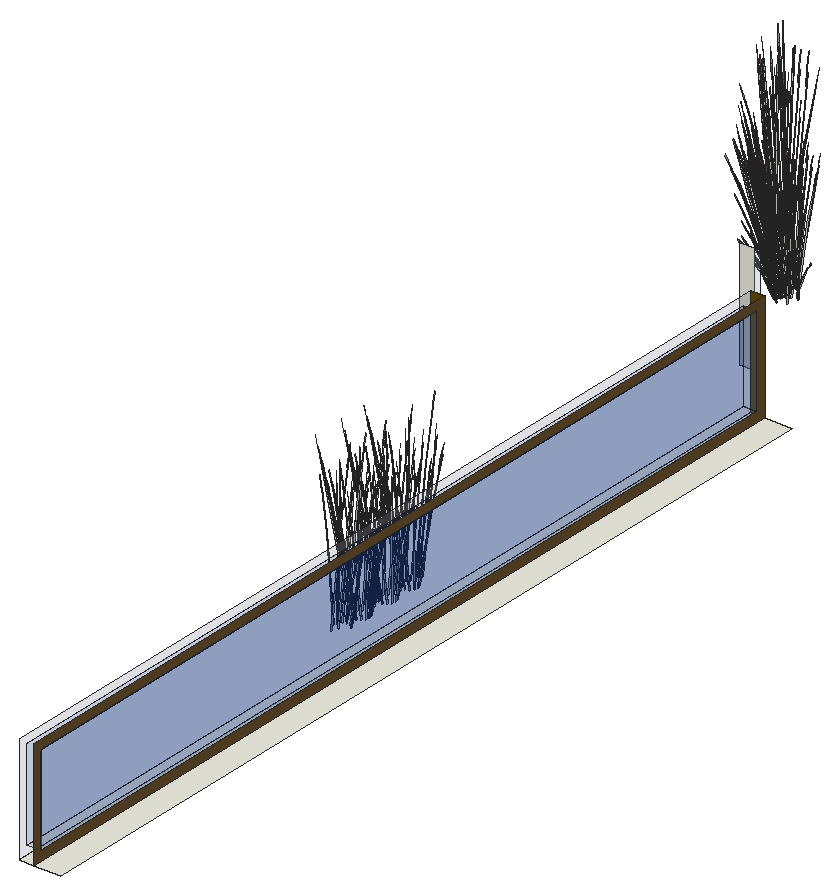
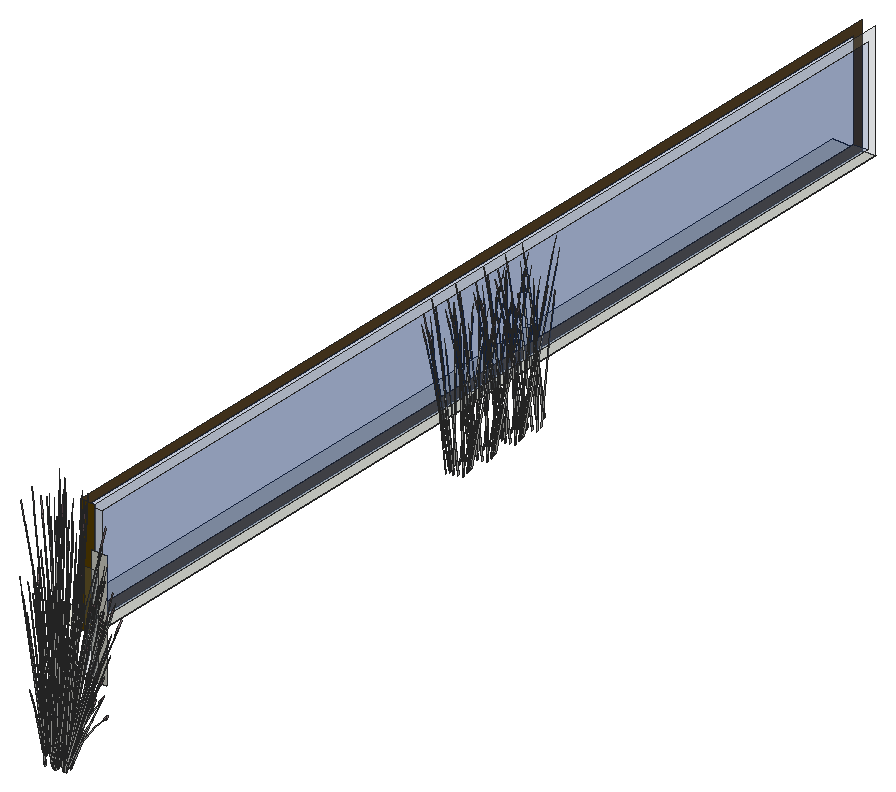
# SketchUp Ruby script. Lengths in inches.
U = 1.inch
M = Sketchup.active_model
def pt(a) = Geom::Point3d.new(a.map { |v| v * U })
def face(e, loops, mat)
  f = e.add_face(loops[0].map { |a| pt(a) })
  loops[1..].each { |l| e.add_face(l.map { |a| pt(a) }).erase! }
  f.material = f.back_material = mat if mat
  f
end
# faces: each face lists its corners as indices into pts; further lists are holes
def faces(e, pts, list, mat = nil) = list.each { |f| face(e, (f[0].is_a?(Array) ? f : [f]).map { |l| l.map { |i| pts[i] } }, mat) }
# xy, xz, yz: faces in a plane at the given z, y or x. An outline is a flat list of corners, or four numbers for a rectangle; further outlines are holes
def ring(l) = l.size == 4 ? [[l[0], l[1]], [l[2], l[1]], [l[2], l[3]], [l[0], l[3]]] : l.each_slice(2).to_a
def flat(e, list, mat, &to3) = list.each { |f| face(e, (f[0].is_a?(Array) ? f : [f]).map { |l| ring(l).map { |u, v| to3.(u, v) } }, mat) }
def xy(e, z, list, mat = nil) = flat(e, list, mat) { |x, y| [x, y, z] }
def xz(e, y, list, mat = nil) = flat(e, list, mat) { |x, z| [x, y, z] }
def yz(e, x, list, mat = nil) = flat(e, list, mat) { |y, z| [x, y, z] }
def lines(e, pts, list) = list.each { |a, b| e.add_line(pt(pts[a]), pt(pts[b])) }
# prism: a flat outline (further loops are holes) pulled along v
def prism(e, loops, v, mat = nil)
  f = face(e, loops, mat); d = Geom::Vector3d.new(v.map { |x| x * U })
  f.pushpull(f.normal.samedirection?(d) ? d.length : -d.length)
end
def box(e, o, s, mat = nil) = prism(e, [[o, [o[0] + s[0], o[1], o[2]], [o[0] + s[0], o[1] + s[1], o[2]], [o[0], o[1] + s[1], o[2]]]], [0, 0, s[2]], mat)
def at(x, y, z, deg = 0) = Geom::Transformation.translation(pt([x, y, z])) * Geom::Transformation.rotation(ORIGIN, Z_AXIS, deg.degrees)
def axes(o, x, y, z) = Geom::Transformation.new([*x, 0, *y, 0, *z, 0, *pt(o).to_a, 1])
def part(name) = M.definitions.add(name)
# library, detail: a bought-in or finely detailed component or shape, given as its bounding box
def library(name, o, s) = part(name).tap { |d| box(d.entities, o, s) }
def detail(e, o, s) = box(e.add_group.entities, o, s)
def put(e, d, t, mat = nil) = e.add_instance(d, t).tap { |i| i.material = mat if mat }
def group(e, t, mat = nil) = e.add_group.tap { |g| g.transformation = t; g.material = mat if mat }.entities
root = M.entities
M.materials.add("D01_Frost_White").color = [238, 238, 227]
M.materials.add("D08_Bronzed_Mustard").color = [102, 74, 0]
M.materials.add("Glass_Basic_01").color = [161, 173, 186]
M.materials["Glass_Basic_01"].alpha = 0.25
M.materials.add("Glass_Sky Reflection_01").color = [0, 46, 142]
M.materials["Glass_Sky Reflection_01"].alpha = 0.25
M.materials.add("LightPink_Translucent").color = [144, 107, 117]
M.materials["LightPink_Translucent"].alpha = 0.75
M.materials.add("Wood_Veneer_15_1K").color = [103, 79, 44]
c1 = part("blade")
p = [[2.15,0.21,22],[0,0.17,0],[0.09,0.45,0],[2.18,0.31,22],[2.29,0.31,22],[0.38,0.45,0],
  [2.48,0.24,33],[2.49,0.24,33],[2.48,0.22,33]]
faces(c1.entities,p,[[0,1,2,3],[4,5,2,3],[6,3,4,7],[8,0,3,6]])
c2 = part("seeds")
p = [[0.3,-0.1,1.38],[-0.01,-0.03,1.59],[-0.01,-0.03,0.03],[0.14,-0.07,-0.07],[0.29,-0.03,3],[0.15,0.01,3.11]]
faces(c2.entities,p,[[0,1,2,3],[1,0,4,5]],"LightPink_Translucent")
c3 = part("blade with seeds")
put(c3.entities,c1,at(0,0,0))
put(c3.entities,c2,axes([2.4,0.25,30.99],[1.5799,-0.05474,1.17369],[-0.12525,1.92788,0.29478],[-0.07173,-0.02425,1.56792]))
xy(root,156,[[439,373,442,574.02],[442,373,448,574.02]],"D01_Frost_White")
xy(root,158,[[439,375,442,572.02]],"Glass_Basic_01")
xz(root,572.02,[[439,158,442,178]],"Glass_Basic_01")
xz(root,574.02,[[439,156,442,180]],"D08_Bronzed_Mustard")
xz(root,586,[[427,156,430,180]],"D01_Frost_White")
xz(root,588,[[427,158,430,178]],"Glass_Basic_01")
yz(root,439,[[[373,156,574.02,180],[375,158,572.02,178]]],"Glass_Basic_01")
yz(root,439,[[375,158,572.02,178]],"Glass_Sky Reflection_01")
yz(root,442,[[375,158,572.02,178]],"Glass_Sky Reflection_01")
yz(root,442,[[[373,156,574.02,180],[375,158,572.02,178]]],"Wood_Veneer_15_1K")
put(root,c3,axes([429.26,472.51,154.77],[0.28319,-0.27058,-0.05481],[0.25948,0.29635,-0.2485],[0.01827,0.08397,0.81966]))
put(root,c3,axes([428.77,471.52,154.28],[-0.4038,-0.12331,0.45013],[0.13808,-0.40538,0.37115],[0.02427,0.15942,0.93144]))
put(root,c3,axes([427.46,473.45,154.27],[0.34057,0.13158,0.29918],[-0.09933,0.38387,-0.38624],[-0.13712,0.0352,0.73904]))
put(root,c3,axes([428.4,477.19,154.3],[0.45651,-0.12123,0.45419],[0.07923,0.47555,0.3745],[-0.10736,-0.14016,0.93983]))
put(root,c3,axes([430.36,474.97,154.27],[-0.23317,-0.29531,0.29918],[0.26625,-0.27955,-0.38624],[0.13527,0.04253,0.73904]))
put(root,c3,axes([429.43,477.58,154.27],[-0.12355,0.36271,0.29918],[-0.36044,-0.10579,-0.38624],[-0.03305,-0.14603,0.73904]))
put(root,c3,axes([430.21,477.99,154.27],[-0.27728,0.24833,0.29918],[-0.26248,-0.28355,-0.38624],[0.03994,-0.14407,0.73904]))
put(root,c3,axes([427.52,474.37,154.27],[0.35672,-0.06741,0.29918],[0.09419,0.38534,-0.38624],[-0.10222,0.1035,0.73904]))
put(root,c3,axes([428.56,477.64,154.27],[0.06329,0.37991,0.29918],[-0.36182,0.10032,-0.38624],[-0.09718,-0.10887,0.73904]))
put(root,c3,axes([427.48,477.89,154.3],[0.33843,-0.34808,0.45419],[0.29188,0.36965,0.3745],[-0.15878,-0.06421,0.93983]))
put(root,c3,axes([426.71,475.46,154.77],[0.36162,0.1259,-0.05481],[-0.11124,0.3875,-0.2485],[-0.05915,0.05883,0.81966]))
put(root,c3,axes([429.64,475.48,154.27],[-0.06329,-0.37991,0.29918],[0.36182,-0.10032,-0.38624],[0.09718,0.10887,0.73904]))
put(root,c3,axes([430.6875,478.76,154.27],[-0.35672,0.06741,0.29918],[-0.09419,-0.38534,-0.38624],[0.10222,-0.1035,0.73904]))
put(root,c3,axes([428,475.14,154.27],[0.27728,-0.24833,0.29918],[0.26248,0.28355,-0.38624],[-0.03994,0.14407,0.73904]))
put(root,c3,axes([428.78,475.54,154.27],[0.12355,-0.36271,0.29918],[0.36044,0.10579,-0.38624],[0.03305,0.14603,0.73904]))
put(root,c3,axes([427.84,478.15,154.27],[0.23317,0.29531,0.29918],[-0.26625,0.27955,-0.38624],[-0.13527,-0.04253,0.73904]))
put(root,c3,axes([429.26,476.84,154.77],[0.28319,-0.27058,-0.05481],[0.25948,0.29635,-0.2485],[0.01827,0.08397,0.81966]))
put(root,c3,axes([428.77,475.84,154.28],[-0.4038,-0.12331,0.45013],[0.13808,-0.40538,0.37115],[0.02427,0.15942,0.93144]))
put(root,c3,axes([430.75,479.68,154.27],[-0.34057,-0.13158,0.29918],[0.09933,-0.38387,-0.38624],[0.13712,-0.0352,0.73904]))
put(root,c3,axes([427.46,478.98,154.27],[0.34057,0.13158,0.29918],[-0.09933,0.38387,-0.38624],[-0.13712,0.0352,0.73904]))
put(root,c3,axes([430.36,480.51,154.27],[-0.23317,-0.29531,0.29918],[0.26625,-0.27955,-0.38624],[0.13527,0.04253,0.73904]))
put(root,c3,axes([427.52,479.9,154.27],[0.35672,-0.06741,0.29918],[0.09419,0.38534,-0.38624],[-0.10222,0.1035,0.73904]))
put(root,c3,axes([428.4,484.41,154.3],[0.45651,-0.12123,0.45419],[0.07923,0.47555,0.3745],[-0.10736,-0.14016,0.93983]))
put(root,c3,axes([426.71,481,154.77],[0.36162,0.1259,-0.05481],[-0.11124,0.3875,-0.2485],[-0.05915,0.05883,0.81966]))
put(root,c3,axes([429.64,481.02,154.27],[-0.06329,-0.37991,0.29918],[0.36182,-0.10032,-0.38624],[0.09718,0.10887,0.73904]))
put(root,c3,axes([429.43,484.79,154.27],[-0.12355,0.36271,0.29918],[-0.36044,-0.10579,-0.38624],[-0.03305,-0.14603,0.73904]))
put(root,c3,axes([430.21,485.2,154.27],[-0.27728,0.24833,0.29918],[-0.26248,-0.28355,-0.38624],[0.03994,-0.14407,0.73904]))
put(root,c3,axes([428,480.67,154.27],[0.27728,-0.24833,0.29918],[0.26248,0.28355,-0.38624],[-0.03994,0.14407,0.73904]))
put(root,c3,axes([428.78,481.08,154.27],[0.12355,-0.36271,0.29918],[0.36044,0.10579,-0.38624],[0.03305,0.14603,0.73904]))
put(root,c3,axes([428.56,484.85,154.27],[0.06329,0.37991,0.29918],[-0.36182,0.10032,-0.38624],[-0.09718,-0.10887,0.73904]))
put(root,c3,axes([427.48,485.1,154.3],[0.33843,-0.34808,0.45419],[0.29188,0.36965,0.3745],[-0.15878,-0.06421,0.93983]))
put(root,c3,axes([429.26,482.375,154.77],[0.28319,-0.27058,-0.05481],[0.25948,0.29635,-0.2485],[0.01827,0.08397,0.81966]))
put(root,c3,axes([428.77,481.38,154.28],[-0.4038,-0.12331,0.45013],[0.13808,-0.40538,0.37115],[0.02427,0.15942,0.93144]))
put(root,c3,axes([430.6875,485.97,154.27],[-0.35672,0.06741,0.29918],[-0.09419,-0.38534,-0.38624],[0.10222,-0.1035,0.73904]))
put(root,c3,axes([427.84,485.37,154.27],[0.23317,0.29531,0.29918],[-0.26625,0.27955,-0.38624],[-0.13527,-0.04253,0.73904]))
put(root,c3,axes([430.75,486.89,154.27],[-0.34057,-0.13158,0.29918],[0.09933,-0.38387,-0.38624],[0.13712,-0.0352,0.73904]))
put(root,c3,axes([427.46,486.2,154.27],[0.34057,0.13158,0.29918],[-0.09933,0.38387,-0.38624],[-0.13712,0.0352,0.73904]))
put(root,c3,axes([428.4,490.57,154.3],[0.45651,-0.12123,0.45419],[0.07923,0.47555,0.3745],[-0.10736,-0.14016,0.93983]))
put(root,c3,axes([430.36,487.72,154.27],[-0.23317,-0.29531,0.29918],[0.26625,-0.27955,-0.38624],[0.13527,0.04253,0.73904]))
put(root,c3,axes([429.43,490.96,154.27],[-0.12355,0.36271,0.29918],[-0.36044,-0.10579,-0.38624],[-0.03305,-0.14603,0.73904]))
put(root,c3,axes([427.52,487.12,154.27],[0.35672,-0.06741,0.29918],[0.09419,0.38534,-0.38624],[-0.10222,0.1035,0.73904]))
put(root,c3,axes([430.21,491.37,154.27],[-0.27728,0.24833,0.29918],[-0.26248,-0.28355,-0.38624],[0.03994,-0.14407,0.73904]))
put(root,c3,axes([426.71,488.21,154.77],[0.36162,0.1259,-0.05481],[-0.11124,0.3875,-0.2485],[-0.05915,0.05883,0.81966]))
put(root,c3,axes([428.56,491.02,154.27],[0.06329,0.37991,0.29918],[-0.36182,0.10032,-0.38624],[-0.09718,-0.10887,0.73904]))
put(root,c3,axes([429.64,488.23,154.27],[-0.06329,-0.37991,0.29918],[0.36182,-0.10032,-0.38624],[0.09718,0.10887,0.73904]))
put(root,c3,axes([427.48,491.27,154.3],[0.33843,-0.34808,0.45419],[0.29188,0.36965,0.3745],[-0.15878,-0.06421,0.93983]))
put(root,c3,axes([428,487.89,154.27],[0.27728,-0.24833,0.29918],[0.26248,0.28355,-0.38624],[-0.03994,0.14407,0.73904]))
put(root,c3,axes([430.6875,492.14,154.27],[-0.35672,0.06741,0.29918],[-0.09419,-0.38534,-0.38624],[0.10222,-0.1035,0.73904]))
put(root,c3,axes([428.78,488.29,154.27],[0.12355,-0.36271,0.29918],[0.36044,0.10579,-0.38624],[0.03305,0.14603,0.73904]))
put(root,c3,axes([429.26,489.59,154.77],[0.28319,-0.27058,-0.05481],[0.25948,0.29635,-0.2485],[0.01827,0.08397,0.81966]))
put(root,c3,axes([428.77,488.59,154.28],[-0.4038,-0.12331,0.45013],[0.13808,-0.40538,0.37115],[0.02427,0.15942,0.93144]))
put(root,c3,axes([427.84,491.53,154.27],[0.23317,0.29531,0.29918],[-0.26625,0.27955,-0.38624],[-0.13527,-0.04253,0.73904]))
put(root,c3,axes([430.75,493.06,154.27],[-0.34057,-0.13158,0.29918],[0.09933,-0.38387,-0.38624],[0.13712,-0.0352,0.73904]))
put(root,c3,axes([427.46,492.36,154.27],[0.34057,0.13158,0.29918],[-0.09933,0.38387,-0.38624],[-0.13712,0.0352,0.73904]))
put(root,c3,axes([430.36,493.89,154.27],[-0.23317,-0.29531,0.29918],[0.26625,-0.27955,-0.38624],[0.13527,0.04253,0.73904]))
put(root,c3,axes([427.52,493.28,154.27],[0.35672,-0.06741,0.29918],[0.09419,0.38534,-0.38624],[-0.10222,0.1035,0.73904]))
put(root,c3,axes([426.71,494.38,154.77],[0.36162,0.1259,-0.05481],[-0.11124,0.3875,-0.2485],[-0.05915,0.05883,0.81966]))
put(root,c3,axes([429.64,494.4,154.27],[-0.06329,-0.37991,0.29918],[0.36182,-0.10032,-0.38624],[0.09718,0.10887,0.73904]))
put(root,c3,axes([428,494.05,154.27],[0.27728,-0.24833,0.29918],[0.26248,0.28355,-0.38624],[-0.03994,0.14407,0.73904]))
put(root,c3,axes([428.78,494.46,154.27],[0.12355,-0.36271,0.29918],[0.36044,0.10579,-0.38624],[0.03305,0.14603,0.73904]))
put(root,c3,axes([429.26,495.75,154.77],[0.28319,-0.27058,-0.05481],[0.25948,0.29635,-0.2485],[0.01827,0.08397,0.81966]))
put(root,c3,axes([428.77,494.76,154.28],[-0.4038,-0.12331,0.45013],[0.13808,-0.40538,0.37115],[0.02427,0.15942,0.93144]))
put(root,c3,axes([416.2,609.51,156.77],[0.09368,0.15143,1.44779],[-0.43286,0.12749,0.11706],[-0.09783,-0.23774,0.61892]))
put(root,c3,axes([416.91,608.5,157.48],[-0.06268,-0.06613,1.47793],[-0.4183,0.04193,-0.23373],[-0.06676,-0.15817,0.11853]))
put(root,c3,axes([417.88,609.29,155.68],[-0.11649,0.09547,1.20808],[-0.34886,-0.1671,-0.25981],[0.06467,-0.20781,0.51652]))
put(root,c3,axes([417.35,609.62,157.7],[-0.19559,-0.38351,-0.60019],[0.40262,-0.21373,0.07243],[-0.04574,-0.1853,0.84903]))
put(root,c3,axes([416.08,609.11,155.68],[-0.02482,0.15429,1.20808],[-0.36278,0.12916,-0.25981],[-0.0848,-0.19943,0.51652]))
put(root,c3,axes([417.02,608.77,154.75],[-0.06874,0.01699,1.48974],[-0.38012,-0.19128,-0.22758],[0.00638,-0.15955,0.25375]))
put(root,c3,axes([418.17,609.99,157.7],[0.01066,-0.43628,-0.60019],[0.44902,0.0293,0.07243],[0.04739,-0.18483,0.84903]))
put(root,c3,axes([418.79,609.3125,157.48],[-0.00396,-0.09387,1.47793],[-0.33411,-0.2713,-0.23373],[0.05166,-0.16446,0.11853]))
put(root,c3,axes([417.39,609.29,157.32],[0.12355,-0.36271,-0.29918],[0.36044,0.10579,0.38624],[-0.03305,-0.14603,0.73904]))
put(root,c3,axes([417.66,609.77,156.77],[-0.0763,0.16212,1.44779],[-0.3201,-0.3355,0.11706],[0.1444,-0.2091,0.61892]))
put(root,c3,axes([418.7,608.97,157.47],[-0.04162,0.03603,1.49853],[-0.40776,-0.12155,-0.1416],[-0.01476,-0.15722,0.26519]))
put(root,c3,axes([417.21,609.54,157.45],[-0.40284,-0.11824,-0.43168],[0.13808,-0.40538,-0.33437],[-0.03694,-0.16321,0.82598]))
put(root,c3,axes([417.46,608.53,155.83],[0.05257,0.27504,0.97034],[-0.29163,-0.15233,0.71294],[0.03138,-0.14083,0.21373]))
put(root,c3,axes([418.08,609.85,157.45],[-0.29336,-0.31691,-0.43168],[0.3099,-0.27755,-0.33437],[0.04464,-0.16102,0.82598]))
put(root,c3,axes([416.49,608.28,157.47],[-0.00765,0.05653,1.49853],[-0.37706,0.20517,-0.1416],[-0.11096,-0.10488,0.26519]))
put(root,c3,axes([416.4,609.29,157.8],[0.45651,-0.12123,0.45419],[0.07923,0.47555,0.3745],[-0.10736,-0.14016,0.93983]))
put(root,c3,axes([417.43,609.375,157.49],[0.4038,0.12331,0.40553],[-0.13808,0.40538,0.33437],[-0.02427,-0.15942,0.83914]))
put(root,c3,axes([417.55,609.52,157.75],[-0.40102,0.2196,-0.10273],[-0.19707,-0.38974,-0.57019],[-0.05291,-0.16424,0.8664]))
put(root,c3,axes([418.38,610.02,157.75],[-0.45039,-0.02337,-0.10273],[0.01231,-0.44247,-0.57019],[0.03129,-0.17041,0.8664]))
put(root,c3,axes([418.35,609.73,157.32],[0.27728,-0.24833,-0.29918],[0.26248,0.28355,0.38624],[0.03994,-0.14407,0.73904]))
put(root,c3,axes([415.96,608.86,155.83],[0.21377,0.16416,0.97034],[-0.31132,0.09868,0.71294],[-0.06661,-0.12616,0.21373]))
put(root,c3,axes([417.54,609.35,157.49],[0.30197,-0.1603,0.05432],[0.1478,0.29231,0.42765],[-0.02916,-0.12885,0.65209]))
put(root,c3,axes([416.47,609.73,157.7],[-0.34944,-0.22798,-0.60019],[0.24834,-0.39949,0.07243],[-0.1266,-0.13612,0.84903]))
put(root,c3,axes([416.35,609.43,157.32],[-0.06329,-0.37991,-0.29918],[0.36182,-0.10032,0.38624],[-0.09718,-0.10887,0.73904]))
put(root,c3,axes([416.51,609.39,157.49],[0.18625,-0.29962,0.05432],[0.26523,0.17444,0.42765],[-0.08575,-0.09606,0.65209]))
put(root,c3,axes([415.79,609.35,154.75],[-0.0397,0.06213,1.48974],[-0.40116,0.13396,-0.22758],[-0.09691,-0.12186,0.25375]))
put(root,c3,axes([415.57,609.98,156.77],[0.15222,0.08126,1.44779],[-0.31502,0.34091,0.11706],[-0.19634,-0.15379,0.61892]))
put(root,c3,axes([418.7,609.58,154.75],[-0.06134,-0.03716,1.48974],[-0.15755,-0.41512,-0.22758],[0.10629,-0.11265,0.25375]))
put(root,c3,axes([417.43,609.67,157.76],[-0.12355,0.36271,0.29918],[-0.36044,-0.10579,-0.38624],[-0.03305,-0.14603,0.73904]))
put(root,c3,axes([416.31,609.74,157.45],[-0.40438,0.11212,-0.43168],[-0.07074,-0.4246,-0.33437],[-0.10862,-0.12168,0.82598]))
put(root,c3,axes([418.35,609.83,157.49],[0.29182,0.32181,0.40553],[-0.3099,0.27755,0.33437],[0.05383,-0.15098,0.83914]))
put(root,c3,axes([416.59,609.36,158.08],[-0.2735,0.45217,-0.11506],[-0.39608,-0.2605,-0.63862],[-0.13768,-0.12775,0.97037]))
put(root,c3,axes([418.46,609.86,157.49],[0.33677,0.02198,0.05432],[-0.00923,0.33185,0.42765],[0.03524,-0.12712,0.65209]))
put(root,c3,axes([418.21,610.08,157.76],[-0.27728,0.24833,0.29918],[-0.26248,-0.28355,-0.38624],[0.03994,-0.14407,0.73904]))
put(root,c3,axes([418.7,610.75,157.7],[0.21406,-0.37215,-0.60019],[0.37511,0.26448,0.07243],[0.12781,-0.13483,0.84903]))
put(root,c3,axes([416.38,609.67,155.5],[-0.25622,-0.47263,0],[0.42866,-0.26357,-0.43598],[0.09763,-0.06003,1.38303]))
put(root,c3,axes([418.6875,610.58,157.45],[-0.10528,-0.43067,-0.43168],[0.39868,-0.07534,-0.33437],[0.11425,-0.11568,0.82598]))
put(root,c3,axes([416.95,609.1,155.29],[-0.28319,0.27058,-0.03288],[-0.25948,-0.29635,-0.1491],[-0.01827,-0.08397,0.4918]))
put(root,c3,axes([415.54,609.23,157.48],[-0.08817,-0.00333,1.47793],[-0.28072,0.33293,-0.23373],[-0.14978,-0.06803,0.11853]))
put(root,c3,axes([418.875,610.89,157.75],[-0.37908,-0.26007,-0.10273],[0.21839,-0.37663,-0.57019],[0.1071,-0.13092,0.8664]))
put(root,c3,axes([417.31,612.31,156.3],[0.35414,0.19019,1.27785],[-0.34693,0.40974,0.50532],[-0.1554,-0.24285,1.07126]))
put(root,c3,axes([416.56,609.74,157.76],[0.06329,0.37991,0.29918],[-0.36182,0.10032,-0.38624],[-0.09718,-0.10887,0.73904]))
put(root,c3,axes([415.46,610.99,155.2],[0,-0.47166,-0.41945],[0.45849,0,0],[0,-0.10742,1.33059]))
put(root,c3,axes([416.73,609.6,155.2],[0.38354,-0.23583,-0.41945],[0.22925,0.42288,0],[0.08735,-0.05371,1.33059]))
put(root,c3,axes([419.01,610.41,155.68],[-0.1464,-0.01397,1.20808],[-0.14998,-0.37477,-0.25981],[0.17985,-0.10602,0.51652]))
put(root,c3,axes([415.48,609.98,157.8],[0.33843,-0.34808,0.45419],[0.29188,0.36965,0.3745],[-0.15878,-0.06421,0.93983]))
put(root,c3,axes([419.81,610.77,157.47],[-0.05353,-0.00358,1.49853],[-0.22227,-0.38383,-0.1416],[0.08926,-0.1262,0.26519]))
put(root,c3,axes([419.18,609.72,155.83],[-0.1365,0.2401,0.97034],[-0.11733,-0.32258,0.71294],[0.11274,-0.08083,0.21373]))
put(root,c3,axes([418.98,610.625,157.32],[0.35672,-0.06741,-0.29918],[0.09419,0.38534,0.38624],[0.10222,-0.1035,0.73904]))
put(root,c3,axes([415.63,609.98,157.49],[0.02064,-0.35866,0.05432],[0.3116,0.00983,0.42765],[-0.11936,-0.03753,0.65209]))
put(root,c3,axes([416.7,611.18,155.36],[0.19883,-0.425,-0.37796],[0.41314,0.20454,0.1819],[0,-0.09797,1.2135]))
put(root,c3,axes([415.51,610.09,157.32],[-0.23317,-0.29531,-0.29918],[0.26625,-0.27955,0.38624],[-0.13527,-0.04253,0.73904]))
put(root,c3,axes([416.89,610.97,155.75],[-0.04775,-0.53819,-0.2458],[0.49736,-0.03254,-0.42242],[0.08758,-0.07169,1.34921]))
put(root,c3,axes([415.65,611,155.21],[0.28606,-0.29428,-0.2617],[0.28606,0.29428,0.2617],[0,-0.09479,1.17405]))
put(root,c3,axes([415.54,609.59,155.29],[-0.11822,0.38513,-0.03288],[-0.36385,-0.11847,-0.1491],[-0.05524,-0.06299,0.4918]))
put(root,c3,axes([418.6875,610.85,157.76],[-0.35672,0.06741,0.29918],[-0.09419,-0.38534,-0.38624],[0.10222,-0.1035,0.73904]))
put(root,c3,axes([416.66,611.54,155.75],[-0.46151,-0.22505,-0.2458],[0.22222,-0.475,-0.42242],[-0.0145,-0.11662,1.34921]))
put(root,c3,axes([415.34,611.35,155.5],[-0.51243,0,0],[0,-0.52715,-0.43598],[0,-0.12006,1.38303]))
put(root,c3,axes([415.43,610.41,155.68],[0.08001,0.13132,1.20808],[-0.18437,0.35694,-0.25981],[-0.18931,-0.08532,0.51652]))
put(root,c3,axes([416.82,609.78,155.21],[0.38233,0.1167,-0.2617],[-0.09626,0.41098,0.2617],[0.07708,-0.04739,1.17405]))
put(root,c3,axes([415.76,610.29,157.7],[-0.40965,-0.01136,-0.60019],[0.02751,-0.47821,0.07243],[-0.17355,-0.05047,0.84903]))
put(root,c3,axes([419.01,610.79,157.49],[0.28133,0.19836,0.05432],[-0.16379,0.28248,0.42765],[0.0902,-0.09132,0.65209]))
put(root,c3,axes([418.93,610.71,157.49],[0.10163,0.43409,0.40553],[-0.39868,0.07534,0.33437],[0.1175,-0.10209,0.83914]))
put(root,c3,axes([420.01,611.23,157.48],[0.05687,-0.07184,1.47793],[-0.07279,-0.44069,-0.23373],[0.14268,-0.08356,0.11853]))
put(root,c3,axes([415.74,611.21,155.46],[-0.38118,0.39654,0.25983],[-0.38142,-0.39237,-0.30828],[-0.01331,-0.11261,1.39295]))
put(root,c3,axes([415.2,609.51,157.47],[0.03038,0.04707,1.49853],[-0.14646,0.42312,-0.1416],[-0.14833,0.00306,0.26519]))
put(root,c3,axes([416.95,611.39,155.55],[0.46174,0.2286,0.2033],[-0.22222,0.475,0.42242],[0,-0.1095,1.35626]))
put(root,c3,axes([416.77,612.04,155.55],[0.10862,-0.55889,-0.19793],[0.515,0.09742,0.43313],[-0.08999,-0.07718,1.32161]))
put(root,c3,axes([415.625,610.39,157.45],[-0.29757,0.31243,-0.43168],[-0.2606,-0.33005,-0.33437],[-0.15119,-0.04754,0.82598]))
put(root,c3,axes([415.84,610.25,157.76],[0.23317,0.29531,0.29918],[-0.26625,0.27955,-0.38624],[-0.13527,-0.04253,0.73904]))
put(root,c3,axes([414.95,610.8,155.83],[0.26163,-0.03375,0.97034],[-0.16596,0.29737,0.71294],[-0.12929,-0.04461,0.21373]))
put(root,c3,axes([416.8,611.08,155.79],[-0.44501,0.02912,0.37796],[-0.04024,-0.48332,-0.1819],[0.07967,-0.04899,1.2135]))
put(root,c3,axes([415.78,610.06,157.75],[-0.02194,0.47967,-0.10273],[-0.41546,-0.01311,-0.57019],[-0.16001,-0.03332,0.8664]))
put(root,c3,axes([415.65,611.43,155.59],[0,0.47166,0.41945],[-0.45849,0,0],[0,-0.10742,1.33059]))
put(root,c3,axes([418.89,611.9,157.75],[-0.20619,-0.42709,-0.10273],[0.36595,-0.20988,-0.57019],[0.15422,-0.05635,0.8664]))
put(root,c3,axes([418.87,611.53,157.45],[0.11102,-0.42903,-0.43168],[0.38064,0.14706,-0.33437],[0.15325,-0.03934,0.82598]))
put(root,c3,axes([418.27,609.79,155.5],[0.25622,-0.47263,0],[0.42866,0.26357,-0.43598],[0.09763,0.06003,1.38303]))
put(root,c3,axes([415.25,610.72,156.77],[0.16998,-0.01068,1.44779],[-0.11276,0.46299,0.11706],[-0.24224,-0.02864,0.61892]))
put(root,c3,axes([416.74,611.81,155.36],[-0.24618,-0.39589,-0.37796],[0.37289,-0.27878,0.1819],[-0.07967,-0.04899,1.2135]))
put(root,c3,axes([416.79,611.25,155.49],[0.17817,0.52741,0.38653],[-0.50909,0.1834,0.15168],[0.00622,-0.09691,1.34202]))
put(root,c3,axes([419.28,611.66,155.17],[-0.26394,0.0566,1.1961],[-0.04201,-0.45055,0.06846],[0.18486,-0.06819,0.68062]))
put(root,c3,axes([419.76,611.26,155.4],[-0.25407,-0.3016,-0.05481],[0.27826,-0.27635,-0.2485],[0.07884,-0.01946,0.81966]))
put(root,c3,axes([416.7,611.67,155.79],[-0.19883,0.425,0.37796],[-0.41314,-0.20454,-0.1819],[0,-0.09797,1.2135]))
put(root,c3,axes([417.43,611.3,155.36],[0,-0.54574,0],[0.51243,0,0],[0,0,1.51605]))
put(root,c3,axes([418.05,610.03,155.59],[-0.38354,-0.23583,0.41945],[0.22925,-0.42288,0],[0.08735,0.05371,1.33059]))
put(root,c3,axes([418.8,611.69,157.7],[0.3601,-0.20831,-0.60019],[0.20068,0.4288,0.07243],[0.17399,-0.04871,0.84903]))
put(root,c3,axes([417.18,610.95,155.49],[-0.33979,0.42804,0.38653],[-0.40368,-0.37784,0.15168],[0.08192,-0.04272,1.34202]))
put(root,c3,axes([417.56,611.72,155.43],[-0.38118,-0.40596,-0.0518],[0.38142,-0.40621,0],[-0.01331,-0.01418,1.48322]))
put(root,c3,axes([416.59,610.25,155.58],[-0.11838,0.46875,0.14904],[-0.43321,-0.13265,0.29641],[0.07483,-0.00228,1.35512]))
put(root,c3,axes([418.75,611.77,157.76],[-0.34057,-0.13158,0.29918],[0.09933,-0.38387,-0.38624],[0.13712,-0.0352,0.73904]))
put(root,c3,axes([415.18,611.07,157.49],[0.11578,-0.43006,0.40553],[0.38064,0.14706,0.33437],[-0.14969,0.02584,0.83914]))
put(root,c3,axes([416.42,610.625,154.84],[-0.40337,0.18883,1.08919],[-0.12839,-0.54182,0.42321],[0.24769,0.00901,1.23883]))
put(root,c3,axes([417.5,610.77,155.7],[0.07906,-0.42093,0.12232],[0.38625,0.07307,-0.3493],[0.07029,0.04322,1.07074]))
put(root,c3,axes([415.15,610.96,157.49],[-0.15051,-0.3216,0.05432],[0.27447,-0.15741,0.42765],[-0.12099,0.03106,0.65209]))
